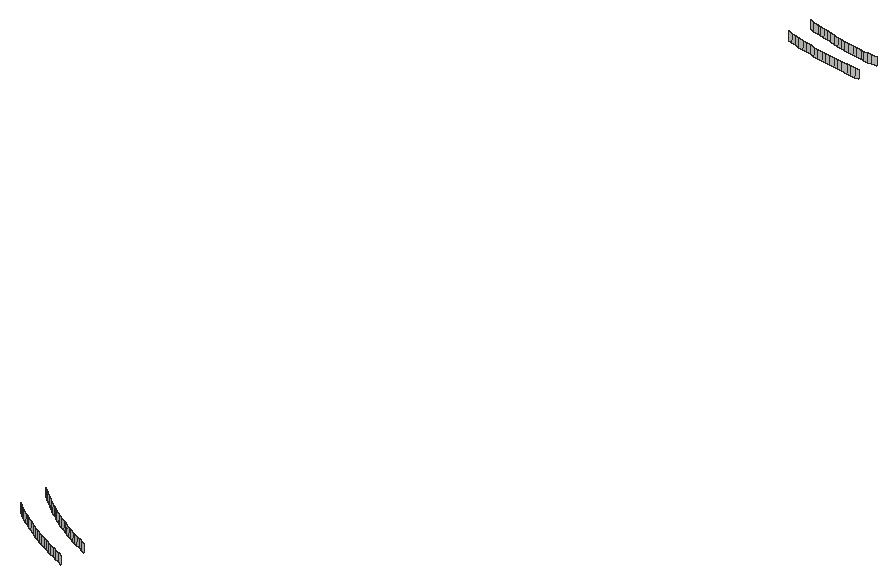
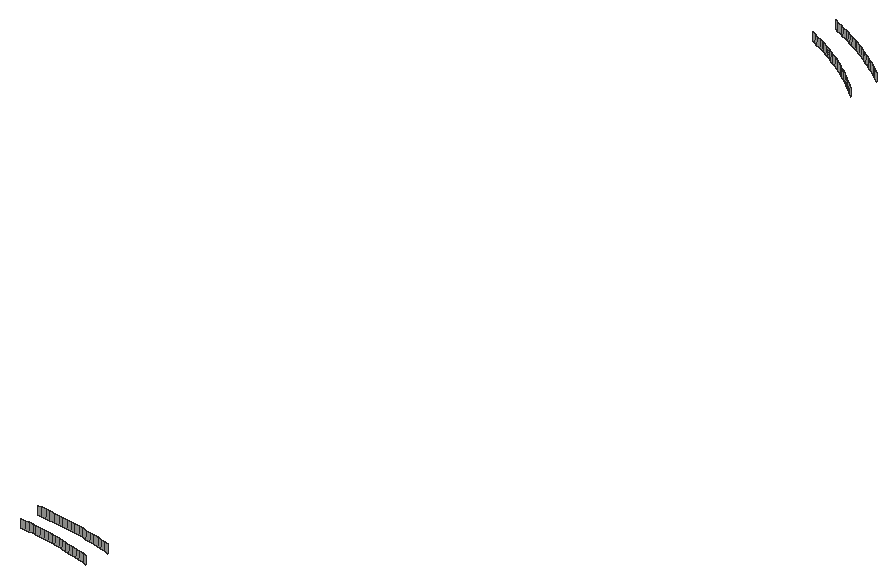
# SketchUp Ruby script. Lengths in inches.
U = 1.inch
M = Sketchup.active_model
def pt(a) = Geom::Point3d.new(a.map { |v| v * U })
def face(e, loops, mat)
  f = e.add_face(loops[0].map { |a| pt(a) })
  loops[1..].each { |l| e.add_face(l.map { |a| pt(a) }).erase! }
  f.material = f.back_material = mat if mat
  f
end
# faces: each face lists its corners as indices into pts; further lists are holes
def faces(e, pts, list, mat = nil) = list.each { |f| face(e, (f[0].is_a?(Array) ? f : [f]).map { |l| l.map { |i| pts[i] } }, mat) }
# xy, xz, yz: faces in a plane at the given z, y or x. An outline is a flat list of corners, or four numbers for a rectangle; further outlines are holes
def ring(l) = l.size == 4 ? [[l[0], l[1]], [l[2], l[1]], [l[2], l[3]], [l[0], l[3]]] : l.each_slice(2).to_a
def flat(e, list, mat, &to3) = list.each { |f| face(e, (f[0].is_a?(Array) ? f : [f]).map { |l| ring(l).map { |u, v| to3.(u, v) } }, mat) }
def xy(e, z, list, mat = nil) = flat(e, list, mat) { |x, y| [x, y, z] }
def xz(e, y, list, mat = nil) = flat(e, list, mat) { |x, z| [x, y, z] }
def yz(e, x, list, mat = nil) = flat(e, list, mat) { |y, z| [x, y, z] }
def lines(e, pts, list) = list.each { |a, b| e.add_line(pt(pts[a]), pt(pts[b])) }
# prism: a flat outline (further loops are holes) pulled along v
def prism(e, loops, v, mat = nil)
  f = face(e, loops, mat); d = Geom::Vector3d.new(v.map { |x| x * U })
  f.pushpull(f.normal.samedirection?(d) ? d.length : -d.length)
end
def box(e, o, s, mat = nil) = prism(e, [[o, [o[0] + s[0], o[1], o[2]], [o[0] + s[0], o[1] + s[1], o[2]], [o[0], o[1] + s[1], o[2]]]], [0, 0, s[2]], mat)
def at(x, y, z, deg = 0) = Geom::Transformation.translation(pt([x, y, z])) * Geom::Transformation.rotation(ORIGIN, Z_AXIS, deg.degrees)
def axes(o, x, y, z) = Geom::Transformation.new([*x, 0, *y, 0, *z, 0, *pt(o).to_a, 1])
def part(name) = M.definitions.add(name)
# library, detail: a bought-in or finely detailed component or shape, given as its bounding box
def library(name, o, s) = part(name).tap { |d| box(d.entities, o, s) }
def detail(e, o, s) = box(e.add_group.entities, o, s)
def put(e, d, t, mat = nil) = e.add_instance(d, t).tap { |i| i.material = mat if mat }
def group(e, t, mat = nil) = e.add_group.tap { |g| g.transformation = t; g.material = mat if mat }.entities
root = M.entities
p = [[150.35,125.52,116],[150.11,125.625,116],[150.11,125.625,116.5],[150.35,125.52,116.5],[149.87,125.73,116],[149.87,125.73,116.5],
  [149.625,125.84,116],[149.625,125.84,116.5],[149.39,125.95,116],[149.39,125.95,116.5],[149.15,126.0625,116],[149.15,126.0625,116.5],
  [148.92,126.18,116],[148.92,126.18,116.5],[148.6875,126.3,116],[148.6875,126.3,116.5],[148.46,126.42,116],[148.46,126.42,116.5],
  [148.23,126.55,116],[148.23,126.55,116.5],[148,126.68,116],[148,126.68,116.5],[147.77,126.8125,116],[147.77,126.8125,116.5],
  [147.55,126.95,116],[147.55,126.95,116.5],[147.33,127.09,116],[147.33,127.09,116.5],[147.11,127.23,116],[147.11,127.23,116.5],
  [150.25,127.2,116],[150.48,127.1,116],[150.48,127.1,116.5],[150.25,127.2,116.5],[146.89,127.37,116],[146.89,127.37,116.5],
  [150.04,127.3,116],[150.04,127.3,116.5],[149.82,127.41,116],[149.82,127.41,116.5],[146.67,127.52,116],[146.67,127.52,116.5],
  [149.6,127.52,116],[149.6,127.52,116.5],[146.46,127.67,116],[146.46,127.67,116.5],[149.39,127.63,116],[149.39,127.63,116.5],
  [149.17,127.74,116],[149.17,127.74,116.5],[146.24,127.82,116],[146.24,127.82,116.5],[148.96,127.86,116],[148.96,127.86,116.5],
  [146.03,127.97,116],[146.03,127.97,116.5],[148.75,127.98,116],[148.75,127.98,116.5],[145.82,128.13,116],[145.82,128.13,116.5],
  [148.54,128.1,116],[148.54,128.1,116.5],[145.62,128.29,116],[145.62,128.29,116.5],[148.33,128.23,116],[148.33,128.23,116.5],
  [148.13,128.35,116],[148.13,128.35,116.5],[147.92,128.48,116],[147.92,128.48,116.5],[147.72,128.62,116],[147.72,128.62,116.5],
  [147.52,128.75,116],[147.52,128.75,116.5],[147.32,128.89,116],[147.32,128.89,116.5],[147.125,129.03,116],[147.125,129.03,116.5],
  [146.93,129.18,116],[146.93,129.18,116.5],[146.74,129.32,116],[146.74,129.32,116.5],[146.55,129.47,116],[146.55,129.47,116.5],
  [146.36,129.62,116],[146.36,129.62,116.5],[146.17,129.78,116],[146.17,129.78,116.5],[145.99,129.93,116],[145.99,129.93,116.5],
  [145.8,130.09,116],[145.8,130.09,116.5],[145.62,130.25,116],[145.62,130.25,116.5],[150.58,186.54,116],[150.3,186.5625,116],
  [150.3,186.5625,116.5],[150.58,186.54,116.5],[149.45,186.64,116],[149.17,186.67,116],[149.17,186.67,116.5],[149.45,186.64,116.5],
  [149.73,186.61,116],[149.73,186.61,116.5],[150.01,186.58,116],[150.01,186.58,116.5],[148.6,186.75,116],[148.32,186.79,116],
  [148.32,186.79,116.5],[148.6,186.75,116.5],[148.89,186.71,116],[148.89,186.71,116.5],[148.04,186.84,116],[147.76,186.88,116],
  [147.76,186.88,116.5],[148.04,186.84,116.5],[147.49,186.9375,116],[147.21,186.99,116],[147.21,186.99,116.5],[147.49,186.9375,116.5],
  [146.93,187.05,116],[146.93,187.05,116.5],[146.65,187.12,116],[146.375,187.18,116],[146.375,187.18,116.5],[146.65,187.12,116.5],
  [146.1,187.25,116],[146.1,187.25,116.5],[145.83,187.33,116],[145.55,187.4,116],[145.55,187.4,116.5],[145.83,187.33,116.5],
  [149.35,188.16,116],[149.61,188.13,116],[149.61,188.13,116.5],[149.35,188.16,116.5],[149.875,188.1,116],[149.875,188.1,116.5],
  [150.14,188.08,116],[150.14,188.08,116.5],[150.41,188.06,116],[150.41,188.06,116.5],[148.56,188.27,116],[148.82,188.23,116],
  [148.82,188.23,116.5],[148.56,188.27,116.5],[149.08,188.19,116],[149.08,188.19,116.5],[148.03,188.36,116],[148.3,188.3125,116],
  [148.3,188.3125,116.5],[148.03,188.36,116.5],[147.51,188.46,116],[147.77,188.41,116],[147.77,188.41,116.5],[147.51,188.46,116.5],
  [146.99,188.58,116],[147.25,188.52,116],[147.25,188.52,116.5],[146.99,188.58,116.5],[146.48,188.7,116],[146.74,188.64,116],
  [146.74,188.64,116.5],[146.48,188.7,116.5],[146.22,188.77,116],[146.22,188.77,116.5],[145.71,188.92,116],[145.96,188.84,116],
  [145.96,188.84,116.5],[145.71,188.92,116.5]]
faces(root,p,[[0,1,2,3],[1,4,5,2],[4,6,7,5],[6,8,9,7],[8,10,11,9],[10,12,13,11],[12,14,15,13],[14,16,17,15],
  [16,18,19,17],[18,20,21,19],[20,22,23,21],[22,24,25,23],[24,26,27,25],[26,28,29,27],[30,31,32,33],[28,34,35,29],
  [36,30,33,37],[38,36,37,39],[34,40,41,35],[42,38,39,43],[40,44,45,41],[46,42,43,47],[48,46,47,49],[44,50,51,45],
  [52,48,49,53],[50,54,55,51],[56,52,53,57],[54,58,59,55],[60,56,57,61],[58,62,63,59],[64,60,61,65],[66,64,65,67],
  [68,66,67,69],[70,68,69,71],[72,70,71,73],[74,72,73,75],[76,74,75,77],[78,76,77,79],[80,78,79,81],[82,80,81,83],
  [84,82,83,85],[86,84,85,87],[88,86,87,89],[90,88,89,91],[92,90,91,93],[94,95,96,97],[98,99,100,101],[102,98,101,103],
  [104,102,103,105],[95,104,105,96],[106,107,108,109],[110,106,109,111],[99,110,111,100],[112,113,114,115],[107,112,115,108],[116,117,118,119],
  [113,116,119,114],[117,120,121,118],[122,123,124,125],[120,122,125,121],[123,126,127,124],[128,129,130,131],[126,128,131,127],[132,133,134,135],
  [133,136,137,134],[136,138,139,137],[138,140,141,139],[142,143,144,145],[143,146,147,144],[146,132,135,147],[148,149,150,151],[149,142,145,150],
  [152,153,154,155],[153,148,151,154],[156,157,158,159],[157,152,155,158],[160,161,162,163],[161,156,159,162],[164,160,163,165],[166,167,168,169],
  [167,164,165,168]])
